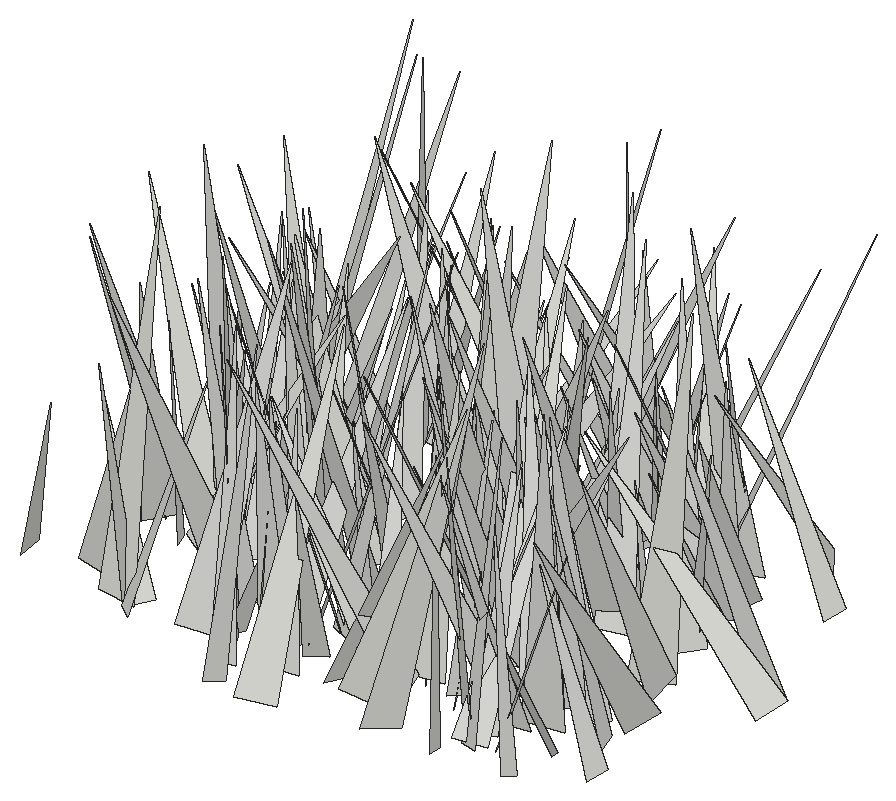
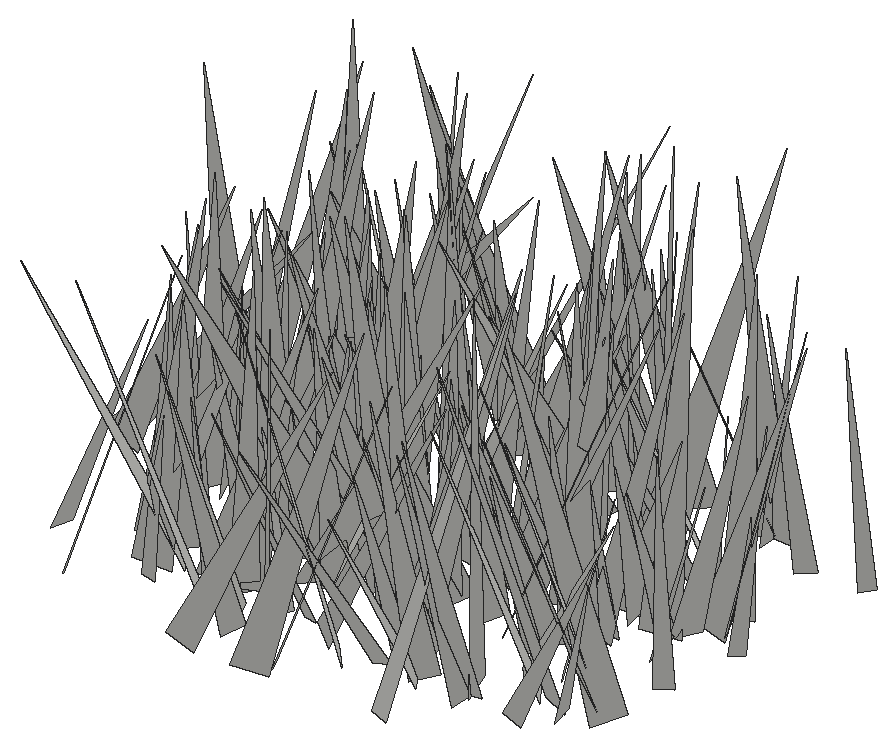
# SketchUp Ruby script. Lengths in inches.
U = 1.inch
M = Sketchup.active_model
def pt(a) = Geom::Point3d.new(a.map { |v| v * U })
def face(e, loops, mat)
  f = e.add_face(loops[0].map { |a| pt(a) })
  loops[1..].each { |l| e.add_face(l.map { |a| pt(a) }).erase! }
  f.material = f.back_material = mat if mat
  f
end
# faces: each face lists its corners as indices into pts; further lists are holes
def faces(e, pts, list, mat = nil) = list.each { |f| face(e, (f[0].is_a?(Array) ? f : [f]).map { |l| l.map { |i| pts[i] } }, mat) }
# xy, xz, yz: faces in a plane at the given z, y or x. An outline is a flat list of corners, or four numbers for a rectangle; further outlines are holes
def ring(l) = l.size == 4 ? [[l[0], l[1]], [l[2], l[1]], [l[2], l[3]], [l[0], l[3]]] : l.each_slice(2).to_a
def flat(e, list, mat, &to3) = list.each { |f| face(e, (f[0].is_a?(Array) ? f : [f]).map { |l| ring(l).map { |u, v| to3.(u, v) } }, mat) }
def xy(e, z, list, mat = nil) = flat(e, list, mat) { |x, y| [x, y, z] }
def xz(e, y, list, mat = nil) = flat(e, list, mat) { |x, z| [x, y, z] }
def yz(e, x, list, mat = nil) = flat(e, list, mat) { |y, z| [x, y, z] }
def lines(e, pts, list) = list.each { |a, b| e.add_line(pt(pts[a]), pt(pts[b])) }
# prism: a flat outline (further loops are holes) pulled along v
def prism(e, loops, v, mat = nil)
  f = face(e, loops, mat); d = Geom::Vector3d.new(v.map { |x| x * U })
  f.pushpull(f.normal.samedirection?(d) ? d.length : -d.length)
end
def box(e, o, s, mat = nil) = prism(e, [[o, [o[0] + s[0], o[1], o[2]], [o[0] + s[0], o[1] + s[1], o[2]], [o[0], o[1] + s[1], o[2]]]], [0, 0, s[2]], mat)
def at(x, y, z, deg = 0) = Geom::Transformation.translation(pt([x, y, z])) * Geom::Transformation.rotation(ORIGIN, Z_AXIS, deg.degrees)
def axes(o, x, y, z) = Geom::Transformation.new([*x, 0, *y, 0, *z, 0, *pt(o).to_a, 1])
def part(name) = M.definitions.add(name)
# library, detail: a bought-in or finely detailed component or shape, given as its bounding box
def library(name, o, s) = part(name).tap { |d| box(d.entities, o, s) }
def detail(e, o, s) = box(e.add_group.entities, o, s)
def put(e, d, t, mat = nil) = e.add_instance(d, t).tap { |i| i.material = mat if mat }
def group(e, t, mat = nil) = e.add_group.tap { |g| g.transformation = t; g.material = mat if mat }.entities
root = M.entities
c1 = part("fur_instance\#9")
p = [[0.8125,0,1.79],[0.67,-0.02,1.48],[0,-0.11,0],[0,0.11,0]]
faces(c1.entities,p,[[0,1,2,3]])
put(root,c1,axes([121.75,413.82,-27.1],[1.49133,-6.04191,1.54576],[-6.23212,-1.50337,0.13646],[-0.23383,1.53405,6.22175]))
put(root,c1,axes([127.07,414.8,-27.1],[-7.35388,-1.92649,0.06127],[-1.88282,7.23164,1.39751],[0.41243,-1.33667,7.47248]))
put(root,c1,axes([123.36,410.6,-27.1],[-3.83392,6.10516,1.11787],[5.9137,3.99214,-1.52073],[1.88436,-0.10697,7.04694]))
put(root,c1,axes([114.97,413.87,-27.1],[-4.71927,-1.33587,1.95814],[-1.09743,5.09822,0.83318],[2.10107,-0.33763,4.83341]))
put(root,c1,axes([122.98,414.57,-27.1],[2.32528,-3.90872,0.2043],[-3.90658,-2.33236,-0.15975],[-0.24182,0.09371,4.54527]))
put(root,c1,axes([130.97,415.68,-27.1],[-7.04471,-1.4589,1.32068],[-0.96261,6.83613,2.41686],[1.71638,-2.15394,6.77607]))
put(root,c1,axes([130.64,411.8125,-27.1],[-5.01766,-1.40088,1.70753],[-1.93126,4.83928,-1.7049],[1.07162,2.16194,4.92267]))
put(root,c1,axes([109.97,414.36,-27.1],[4.41728,-0.60705,0.29796],[-0.51929,-4.30631,-1.07505],[-0.43316,-1.02804,4.32726]))
put(root,c1,axes([121.25,410.86,-27.1],[-5.97598,0.81352,1.54005],[0.17172,5.75229,-2.37225],[1.73323,2.235,5.54496]))
put(root,c1,axes([121.75,414.43,-27.1],[4.45698,-3.93649,1.376],[-3.92382,-4.64074,-0.56675],[-1.41173,0.47074,5.91941]))
put(root,c1,axes([128.1,411.89,-27.1],[7.25129,-2.23194,2.73946],[-2.93898,-7.28136,1.84704],[-1.96177,2.6585,7.35875]))
put(root,c1,axes([121.08,413.58,-27.1],[4.15437,2.45212,1.76514],[2.75663,-4.30471,-0.50784],[-1.23677,-1.35794,4.79727]))
put(root,c1,axes([126.07,413.14,-27.1],[3.27115,-5.93629,2.22387],[-6.24966,-2.60094,2.25],[1.06155,2.98013,6.39355]))
put(root,c1,axes([118,416.32,-27.1],[3.07442,-7.15508,0.96712],[-6.88437,-3.22185,-1.95131],[-2.1762,0.08396,7.5392]))
put(root,c1,axes([122.84,412.96,-27.1],[-0.37436,4.96388,1.61425],[5.21969,0.34743,0.14211],[-0.02763,-1.62026,4.97594]))
put(root,c1,axes([132.09,413.77,-27.1],[4.65437,1.55789,0.49043],[1.62302,-4.57734,-0.86283],[-0.1826,-0.97553,4.83174]))
put(root,c1,axes([136.32,414.03,-27.1],[-4.20728,0.83557,0.99678],[1.00115,4.23485,0.67581],[0.83033,-0.87227,4.23588]))
put(root,c1,axes([130.74,413.6,-27.1],[3.92843,5.06138,3.38638],[5.5366,-4.64662,0.52215],[-2.53598,-2.30413,6.38572]))
put(root,c1,axes([120.65,412.1,-27.1],[0.64289,6.12986,1.03372],[6.0316,-0.86662,1.38779],[-1.50455,-0.85491,6.00521]))
put(root,c1,axes([133.84,412.05,-27.1],[-4.92435,-0.05312,0.24709],[-0.15186,4.47527,-2.06445],[0.20202,2.06935,4.47102]))
put(root,c1,axes([119.71,414.01,-27.1],[4.16125,-1.09144,0.28201],[-1.11074,-4.15389,0.31328],[-0.19241,0.37504,4.29058]))
put(root,c1,axes([112.49,414.71,-27.1],[0.76926,-4.66703,1.07076],[-4.59745,-0.41678,1.48633],[1.33832,1.25083,4.49041]))
put(root,c1,axes([126.06,414.55,-27.1],[-4.18794,0.93567,0.33129],[0.9893,4.05153,1.06324],[0.08071,-1.11073,4.15738]))
put(root,c1,axes([124.67,413.74,-27.1],[6.16079,-1.33707,0.34037],[-1.37023,-6.11166,0.79308],[-0.16154,0.84778,6.25413]))
put(root,c1,axes([132.01,415.01,-27.1],[-1.08629,-5.09453,1.21583],[-5.17343,0.84989,-1.06105],[-0.81738,1.39139,5.09985]))
put(root,c1,axes([115.7,413.76,-27.1],[-3.05082,2.35934,0.28628],[2.37608,3.01778,0.45074],[-0.05159,-0.53147,3.83025]))
put(root,c1,axes([114.69,413.4375,-27.1],[0.76042,7.54721,2.45249],[7.93568,-0.724,-0.23253],[-0.00259,-2.46349,7.58186]))
put(root,c1,axes([135.22,418.04,-27.1],[5.40671,-4.03304,0.21931],[-3.53675,-4.90438,-2.9974],[-1.95061,-2.2864,6.04264]))
put(root,c1,axes([119.75,414.11,-27.1],[4.32475,3.25099,2.86901],[3.37923,-5.06616,0.64681],[-2.71679,-1.12634,5.37159]))
put(root,c1,axes([115.56,412.82,-27.1],[2.99735,3.72962,0.28981],[3.68324,-3.00724,0.60693],[-0.65404,0.15682,4.74613]))
put(root,c1,axes([132.59,415.61,-27.1],[2.16747,-6.96935,1.82134],[-7.20329,-2.08612,0.58967],[0.04123,1.91397,7.27476]))
put(root,c1,axes([131.39,412.8,-27.1],[2.56304,5.03632,1.18387],[4.82189,-2.80423,1.49027],[-1.87495,-0.32715,5.45094]))
put(root,c1,axes([118.48,413.36,-27.1],[-2.56408,6.91655,2.55207],[6.94878,3.17004,-1.60986],[2.46298,-1.74312,7.19872]))
put(root,c1,axes([134.1875,414.28,-27.1],[-5.38862,-5.55187,0.24968],[-4.68183,4.34761,-4.37054],[-2.99434,3.19341,6.38427]))
put(root,c1,axes([118.8125,415.65,-27.1],[-6.63003,0.58928,2.6026],[0.94805,7.03587,0.82207],[2.49439,-1.10786,6.6052]))
put(root,c1,axes([131.35,413.7,-27.1],[-4.05743,3.11883,1.27429],[2.94276,4.25195,-1.03673],[1.64046,0.08657,5.0115]))
put(root,c1,axes([126.52,413.87,-27.1],[-2.91757,4.706,0.99504],[4.75363,2.9987,-0.24403],[0.73452,-0.71423,5.53165]))
put(root,c1,axes([129.02,415.02,-27.1],[3.30079,2.00098,0.99665],[2.11543,-3.37049,-0.23912],[-0.72261,-0.72685,3.85253]))
put(root,c1,axes([122.03,417.01,-27.1],[-4.79453,-5.10071,1.01007],[-5.15614,4.84133,-0.02673],[0.67211,0.75447,7.00029]))
put(root,c1,axes([128.05,417.26,-27.1],[5.66121,2.03663,0.41958],[1.99596,-4.98096,-2.75306],[0.58316,-2.72311,5.34956]))
put(root,c1,axes([135.13,416.07,-27.1],[-4.98874,-1.77944,1.14235],[-1.81158,5.1064,0.04294],[1.09068,0.3424,5.29642]))
put(root,c1,axes([131.25,413.07,-27.1],[-3.49002,4.97532,0.38419],[4.70613,3.43753,-1.76559],[1.65943,0.71499,5.81522]))
put(root,c1,axes([116.8,417.63,-27.1],[-4.19902,-6.23031,2.61813],[-6.01537,4.8505,1.89504],[3.08005,0.97931,7.27031]))
put(root,c1,axes([127.11,415.78,-27.1],[-1.46748,5.77462,2.34569],[6.13429,1.76496,-0.50731],[1.10405,-2.13089,5.93652]))
put(root,c1,axes([126.41,416.12,-27.1],[5.41159,0.09186,1.28906],[0.07062,-5.56242,0.09991],[-1.29039,0.08081,5.41145]))
put(root,c1,axes([132.98,417.5,-27.1],[2.11565,-6.08651,1.80009],[-6.2822,-2.27872,-0.32139],[-0.90548,1.58863,6.43571]))
put(root,c1,axes([116.19,417.57,-27.1],[5.48101,-1.25937,0.85366],[-1.15676,-5.52263,-0.72019],[-0.98826,-0.52035,5.57753]))
put(root,c1,axes([116.03,416.14,-27.1],[3.45283,2.51437,0.03768],[2.48973,-3.40925,-0.65094],[0.3531,-0.54815,4.22141]))
put(root,c1,axes([123.1,416.98,-27.1],[-4.21656,2.08304,0.19454],[2.06998,4.09043,1.06765],[-0.30342,-1.04195,4.58024]))
put(root,c1,axes([128.22,418.82,-27.1],[-3.59271,-3.52154,0.36411],[-3.38524,3.56898,1.11534],[1.03633,-0.55007,4.90559]))
put(root,c1,axes([133.88,417.23,-27.1],[1.42768,-3.34431,1.65268],[-3.54003,-1.77266,-0.52903],[-1.17641,1.27565,3.59761]))
put(root,c1,axes([123.36,418.99,-27.1],[-0.67207,-6.04885,0.74296],[-6.03248,0.76649,0.78356],[0.86591,0.6451,6.03542]))
put(root,c1,axes([129.29,418.52,-27.1],[-0.74587,-6.40704,1.23448],[-6.45249,0.53969,-1.09751],[-0.96927,1.33753,6.35625]))
put(root,c1,axes([112.27,419.03,-27.1],[4.76035,-4.27512,0.72339],[-4.20428,-4.81383,-0.78223],[-1.06017,-0.10597,6.35025]))
put(root,c1,axes([134.24,420.4,-27.1],[6.25747,-1.85529,1.59771],[-1.00282,-5.94215,-2.97253],[-2.23363,-2.52972,5.81052]))
put(root,c1,axes([127.14,415.69,-27.1],[5.31118,5.11176,2.74997],[4.78098,-5.96627,1.85658],[-3.29161,-0.41778,7.13385]))
put(root,c1,axes([129.2,416.97,-27.1],[-7.32876,-0.97242,0.83606],[-1.07916,7.29688,-0.97277],[0.69283,1.07947,7.32872]))
put(root,c1,axes([121.81,419.35,-27.1],[-2.25691,-7.5793,1.44794],[-7.71352,2.17504,-0.63772],[-0.20948,1.56823,7.88243]))
put(root,c1,axes([125.21,418.43,-27.1],[-3.55918,-3.90599,0.48478],[-3.91702,3.45103,-0.95229],[-0.38568,0.99656,5.19785]))
put(root,c1,axes([128.62,415.44,-27.1],[1.86893,4.92203,0.04113],[4.36091,-1.67616,2.42774],[-2.28266,0.8277,4.67176]))
put(root,c1,axes([124.77,419.37,-27.1],[4.05285,-0.43746,0.41546],[-0.3233,-3.95717,-1.01285],[-0.50937,-0.96903,3.94856]))
put(root,c1,axes([122.45,418.25,-27.1],[0.90627,3.33198,1.59944],[3.57947,-1.20149,0.47479],[-0.9207,-1.39138,3.42023]))
put(root,c1,axes([112.03,419.77,-27.1],[-5.14482,-3.13912,1.24988],[-3.04737,5.29445,0.7535],[1.4594,-0.01101,5.97959]))
put(root,c1,axes([113.89,418.13,-27.1],[-3.72029,-1.54775,1.40082],[-1.82397,3.80239,-0.64288],[1.01535,1.15959,3.97778]))
put(root,c1,axes([130.78,417.55,-27.1],[-2.14866,5.91991,1.32548],[6.06222,2.04254,0.70466],[-0.22751,-1.48381,6.25824]))
put(root,c1,axes([122.1875,415.27,-27.1],[6.2923,4.31715,0.79405],[3.75537,-6.01297,2.93303],[-2.27277,2.01685,7.04472]))
put(root,c1,axes([118.12,421.52,-27.1],[-1.88375,-7.99896,1.23534],[-7.80751,2.13018,1.88761],[2.13359,0.73274,7.99805]))
put(root,c1,axes([124.57,419.62,-27.1],[4.01557,-5.25956,2.05629],[-5.53772,-4.16187,0.169],[-1.10676,1.74125,6.61508]))
put(root,c1,axes([122.62,416.42,-27.1],[3.92721,6.27569,0.86047],[6.07775,-4.01843,1.56873],[-1.78486,0.12492,7.23508]))
put(root,c1,axes([125.4375,422.11,-27.1],[4.78768,-6.87101,0.53821],[-6.76798,-4.81092,-1.21319],[-1.30189,-0.25808,8.28619]))
put(root,c1,axes([112.44,420.25,-27.1],[-0.64276,-5.9949,1.38637],[-6.03632,0.34404,-1.31091],[-1.1932,1.48889,5.88502]))
put(root,c1,axes([120.71,416.26,-27.1],[-4.56425,4.1816,0.8559],[3.58274,4.43445,-2.55936],[2.31998,1.37862,5.63629]))
put(root,c1,axes([114.54,418.15,-27.1],[2.28513,5.39499,0.34939],[5.12885,-2.04337,-1.99232],[1.70965,-1.08097,5.50984]))
put(root,c1,axes([110.66,420.98,-27.1],[4.01864,-1.00258,0.99057],[-0.63294,-3.95809,-1.43832],[-1.25928,-1.21004,3.88405]))
put(root,c1,axes([119.65,419.21,-27.1],[-6.31517,-2.67121,2.41272],[-3.08957,6.52254,-0.86542],[1.84694,1.77736,6.80204]))
put(root,c1,axes([127.1,419.68,-27.1],[4.74645,-3.63152,0.20608],[-3.44873,-4.38539,2.15263],[1.15614,1.82746,5.57521]))
put(root,c1,axes([119.5,418.17,-27.1],[-6.71,0.21588,0.88951],[-0.0468,6.49159,-1.92847],[0.91413,1.91692,6.43053]))
put(root,c1,axes([116.85,418.74,-27.1],[-1.85743,4.94831,0.92273],[4.99711,1.93095,-0.29602],[0.60509,-0.75691,5.27714]))
put(root,c1,axes([130.01,423.07,-27.1],[2.00321,-7.73932,0.37509],[-7.71802,-2.02729,-0.61059],[-0.68548,0.20889,7.97102]))
put(root,c1,axes([121.49,420.89,-27.1],[1.52564,-3.34819,0.07276],[-3.07421,-1.36842,1.48995],[1.32851,0.67846,3.36423]))
put(root,c1,axes([127.65,420.69,-27.1],[-2.05605,-4.2865,1.82271],[-4.5186,2.31917,0.35698],[1.13077,1.47345,4.74068]))
put(root,c1,axes([113.77,421.5,-27.1],[1.30407,-7.61557,2.3618],[-7.95747,-1.39423,-0.10194],[-0.50366,2.30972,7.72574]))
put(root,c1,axes([133.57,420.59,-27.1],[-3.8242,6.03816,3.67075],[6.53219,4.61268,-0.78232],[2.69524,-2.61192,7.10435]))
put(root,c1,axes([128.375,420.125,-27.1],[2.97809,2.23148,0.68885],[2.24903,-3.04112,0.12836],[-0.62921,-0.30835,3.71915]))
put(root,c1,axes([128.8,418.32,-27.1],[-3.78371,6.02543,0.57396],[5.96039,3.82698,-0.88298],[1.05307,-0.01122,7.05993]))
put(root,c1,axes([138.27,421.67,-27.1],[-5.02457,3.67244,0.21301],[3.24783,4.25941,3.17608],[-1.72736,-2.67378,5.35216]))
put(root,c1,axes([120.51,421.94,-27.1],[-3.95359,-4.39819,1.62013],[-4.4402,4.19331,0.54823],[1.50116,0.81969,5.8885]))
put(root,c1,axes([133.375,420.91,-27.1],[-3.75742,-0.36081,1.22113],[-0.40687,3.94545,-0.08619],[1.20657,0.20686,3.77372]))
put(root,c1,axes([127.06,423.28,-27.1],[1.34944,-6.66989,1.0863],[-6.57389,-1.5523,-1.36482],[-1.56569,0.76902,6.66676]))
put(root,c1,axes([126.93,420.36,-27.1],[-2.07994,4.49979,1.08625],[4.57933,2.1742,-0.23818],[0.67657,-0.88257,4.95151]))
put(root,c1,axes([127.15,423.63,-27.1],[3.45501,-4.88886,0.26504],[-4.85303,-3.46254,-0.60598],[-0.64754,-0.13474,5.95575]))
put(root,c1,axes([112.99,420.98,-27.1],[-5.78073,2.46703,0.60773],[2.49572,5.79658,0.20851],[0.47643,-0.43109,6.28168]))
put(root,c1,axes([120.31,420.96,-27.1],[-1.88222,6.06948,1.49765],[6.0067,1.32242,2.18977],[-1.73238,-2.00921,5.96542]))
put(root,c1,axes([115.4375,423.01,-27.1],[-1.29627,-6.42722,1.30707],[-6.54569,1.18361,-0.67151],[-0.41416,1.4099,6.52216]))
put(root,c1,axes([114.96,422.69,-27.1],[3.94876,4.2171,2.00571],[4.64379,-3.26946,-2.26834],[0.4919,-2.98768,5.31331]))
put(root,c1,axes([118.19,424.88,-27.1],[-6.16351,-3.9605,0.27898],[-3.73191,5.95492,2.08903],[1.35509,-1.6142,7.02213]))
put(root,c1,axes([126.96,423.53,-27.1],[3.0521,-3.8403,0.46149],[-3.78154,-3.08617,-0.67208],[-0.8129,-0.06212,4.85917]))
put(root,c1,axes([115.87,420.93,-27.1],[-2.49681,4.68547,0.3153],[4.52882,2.308,1.56527],[-1.24213,-1.0033,5.07323]))
put(root,c1,axes([137.68,422.41,-27.1],[-0.80032,5.57612,2.90873],[5.9333,-0.30294,2.21326],[-2.08561,-3.00158,5.18026]))
put(root,c1,axes([117.55,421.87,-27.1],[3.71191,-5.65782,4.04126],[-6.28277,-4.69165,-0.79764],[-2.97818,2.84578,6.7196]))
put(root,c1,axes([128.4,420.99,-27.1],[-3.95695,1.67084,0.9926],[1.45221,4.03835,-1.00857],[1.29152,0.5783,4.17516]))
put(root,c1,axes([119.03,422.3125,-27.1],[-7.40149,0.22253,0.007],[0.22253,7.40149,0.00759],[0.00677,-0.0078,7.40483]))
put(root,c1,axes([115.65,423.8,-27.1],[5.14782,-4.26055,1.16689],[-4.27581,-5.25589,-0.32723],[-1.10966,0.4872,6.67423]))
put(root,c1,axes([126.0625,424.35,-27.1],[7.05622,-1.23215,0.51957],[-1.10047,-6.93599,-1.50315],[-0.75967,-1.39725,7.0035]))
put(root,c1,axes([112.97,422.82,-27.1],[-3.79015,-1.11399,0.60809],[-1.15598,3.82064,-0.20588],[0.52388,0.37109,3.9451]))
put(root,c1,axes([132.7,424.11,-27.1],[-1.98967,-4.65459,1.69235],[-4.24096,2.54317,2.00863],[2.55803,0.59592,4.64644]))
put(root,c1,axes([123.68,423.71,-27.1],[0.0585,-4.06465,0.78718],[-4.11626,0.02739,0.44734],[0.44434,0.78888,4.04038]))
put(root,c1,axes([128.87,424.55,-27.1],[-0.89521,-5.51634,1.09126],[-5.41102,1.14576,1.35291],[1.53027,0.82431,5.42227]))
put(root,c1,axes([113.2,421.76,-27.1],[-3.70619,1.07071,1.22273],[0.63141,3.75399,-1.37341],[1.4976,1.06701,3.605]))
put(root,c1,axes([125.53,424.0625,-27.1],[3.59874,-6.83955,3.08177],[-7.12327,-4.18751,-0.97538],[-2.35281,2.21652,7.66674]))
put(root,c1,axes([123.65,423.3,-27.1],[-2.45983,6.23998,3.07468],[6.83629,2.77173,-0.15592],[1.28687,-2.79677,6.7055]))
put(root,c1,axes([111.18,424.52,-27.1],[0.91273,-4.1627,0.50654],[-4.12867,-0.80133,0.85424],[0.734,0.66898,4.1751]))
put(root,c1,axes([115.26,420.78,-27.1],[-5.60466,1.1961,0.32776],[0.92969,5.05609,-2.5538],[0.82084,2.4404,5.13039]))
put(root,c1,axes([122.8125,423.9,-27.1],[7.01983,-0.71592,2.31882],[-0.6287,-7.39114,-0.37866],[-2.34397,-0.1616,7.04608]))
put(root,c1,axes([133.1,426.07,-27.1],[2.61621,-5.42084,0.25429],[-5.22177,-2.59146,-1.52055],[-1.47757,-0.43991,5.82391]))
put(root,c1,axes([134.76,424.09,-27.1],[-1.27388,-3.61865,0.59779],[-3.46584,0.98064,-1.44951],[-1.19998,1.0092,3.55195]))
put(root,c1,axes([122.98,421.62,-27.1],[-0.78819,5.89997,0.04998],[5.7265,0.75282,1.4401],[-1.42105,-0.23877,5.77555]))
put(root,c1,axes([116.57,423.01,-27.1],[-1.7521,4.37342,1.24469],[4.49457,1.86786,-0.23622],[0.6891,-1.06311,4.7054]))
put(root,c1,axes([133.18,423.125,-27.1],[-6.12251,3.37612,2.03098],[3.42132,6.417,-0.35327],[1.95387,-0.65732,6.98272]))
put(root,c1,axes([121.59,424.05,-27.1],[-0.9402,5.50023,2.63792],[6.09336,0.97222,0.14463],[0.28664,-2.62629,5.57814]))
put(root,c1,axes([120.91,423.99,-27.1],[4.20762,-3.32651,0.12048],[-3.15177,-3.91891,1.86887],[1.07075,1.53645,5.02763]))
put(root,c1,axes([127.08,421.95,-27.1],[2.4518,5.85296,0.01413],[5.81055,-2.43218,-0.76857],[0.70347,-0.30989,6.29903]))
put(root,c1,axes([129.95,424.76,-27.1],[-0.88602,-4.48963,1.06047],[-4.46813,0.56653,-1.33464],[-1.14769,1.26043,4.37728]))
put(root,c1,axes([116.01,423.2,-27.1],[4.17653,-0.25853,0.87813],[-0.4857,-4.1025,1.10224],[-0.77592,1.17643,4.03674]))
put(root,c1,axes([132.71,422.75,-27.1],[-5.22043,-0.84385,1.05571],[-1.17009,4.93002,-1.84535],[0.67639,2.01552,4.95577]))
put(root,c1,axes([130.25,422.59,-27.1],[-1.2461,7.24945,1.28302],[7.36015,1.19663,0.38699],[-0.1701,-1.32928,7.34558]))
put(root,c1,axes([126.83,423.125,-27.1],[-3.66348,3.88372,0.60062],[3.90017,3.69385,-0.09601],[0.48235,-0.37054,5.33808]))
put(root,c1,axes([130.51,424.58,-27.1],[4.15283,1.56186,1.94961],[1.7605,-4.5132,-0.13443],[-1.7723,-0.82343,4.43479]))
put(root,c1,axes([132.78,427.03,-27.1],[4.609,-3.3139,0.05026],[-3.15306,-4.41083,-1.68231],[-1.0211,-1.33793,5.42168]))
put(root,c1,axes([131.3,423.52,-27.1],[-1.57636,3.66287,0.67143],[3.67727,1.64614,-0.34684],[0.58749,-0.47537,3.97256]))
put(root,c1,axes([123.48,424.95,-27.1],[4.4628,-4.8312,0.78242],[-4.8199,-4.15484,1.83716],[0.84924,1.80724,6.31521]))
put(root,c1,axes([124.81,424.97,-27.1],[3.82808,-2.96393,0.87418],[-3.08142,-3.76593,0.72521],[-0.23226,1.11183,4.78677]))
put(root,c1,axes([127.22,425.08,-27.1],[3.70956,-2.15387,1.10856],[-2.28011,-3.78925,0.26761],[-0.81802,0.79458,4.28116]))
put(root,c1,axes([121.86,424.77,-27.1],[-3.05036,2.77962,1.08054],[2.93347,3.07501,0.37088],[0.53722,-1.00823,4.11016]))
put(root,c1,axes([131.99,427.41,-27.1],[-3.10911,-5.59083,0.18925],[-5.58666,3.11434,0.22319],[0.28707,0.05678,6.39328]))
put(root,c1,axes([125.95,426.3,-27.1],[-7.5943,2.08618,0.38061],[2.11361,7.33132,1.9887],[-0.17228,-2.01745,7.62041]))
put(root,c1,axes([114.55,426.1,-27.1],[-3.02688,-2.08558,0.64094],[-2.07151,3.09116,0.27563],[0.68504,0.13224,3.66547]))
put(root,c1,axes([111.27,427.59,-27.1],[2.01455,-7.63294,0.11302],[-6.59973,-1.68273,3.99311],[3.83642,1.11337,6.80994]))
put(root,c1,axes([120.86,426.69,-27.1],[-6.83352,3.26319,2.339],[3.80782,6.73136,1.73366],[1.27275,-2.61852,7.37155]))
put(root,c1,axes([128.625,424.63,-27.1],[-5.59489,5.13542,2.2708],[5.22691,5.9344,-0.54239],[2.05147,-1.11455,7.57503]))
put(root,c1,axes([116.65,424.29,-27.1],[5.33264,0.16428,1.51785],[-0.27785,-5.31816,1.55174],[-1.50122,1.56784,5.10452]))
put(root,c1,axes([119.16,424.37,-27.1],[-5.25856,3.05312,1.43062],[2.8843,5.44607,-1.02073],[1.74617,0.1987,5.99435]))
put(root,c1,axes([124.99,426.01,-27.1],[3.66382,-3.28739,1.57998],[-3.52995,-3.75957,0.36325],[-0.918,1.33625,4.90903]))
put(root,c1,axes([127.2,428.11,-27.1],[4.74802,-2.11154,0.82126],[-1.70244,-4.58339,-1.94189],[-1.49491,-1.48682,4.81989]))
put(root,c1,axes([122.82,424.59,-27.1],[1.506,6.6666,0.93752],[6.04421,-0.91584,-3.19677],[2.9648,-1.51928,6.04088]))
put(root,c1,axes([125.47,425.74,-27.1],[-5.46904,-3.01802,0.13387],[-2.92547,5.22183,-1.79189],[-0.75368,1.63119,5.98398]))
put(root,c1,axes([121.11,426.52,-27.1],[0.6303,-6.24139,2.24897],[-6.57772,-0.29373,1.02832],[0.86396,2.31708,6.18828]))
put(root,c1,axes([122.41,425.58,-27.1],[-3.47776,6.78239,3.15196],[7.08859,4.09761,-0.99596],[2.38486,-2.28893,7.55669]))
put(root,c1,axes([128.91,428.3,-27.1],[3.32641,-4.64571,1.36805],[-4.19977,-3.59363,-1.99171],[-2.41165,-0.14974,5.35544]))
put(root,c1,axes([116.39,425.45,-27.1],[-0.0874,4.08723,0.80677],[4.1529,0.14964,-0.30818],[0.33125,-0.79758,4.07653]))
put(root,c1,axes([115.68,426.92,-27.1],[-2.7303,-2.91554,0.15676],[-2.8364,2.59761,-1.08937],[-0.69267,0.85529,3.84294]))
put(root,c1,axes([131.625,427.54,-27.1],[0.51611,-4.80053,1.29544],[-4.96034,-0.40702,0.46794],[0.34389,1.33374,4.80546]))
put(root,c1,axes([123.13,424.66,-27.1],[-3.56356,5.20391,0.71647],[5.00613,3.62664,-1.4419],[1.59144,0.24443,6.14008]))
put(root,c1,axes([125.91,424.35,-27.1],[7.47799,-1.52657,1.95795],[-2.25093,-6.79047,3.30259],[-1.04752,3.69369,6.88067]))
put(root,c1,axes([125.23,428.54,-27.1],[4.19489,0.81761,0.41517],[0.91291,-3.90671,-1.53042],[-0.08632,-1.58339,3.99042]))
put(root,c1,axes([133.32,431.36,-27.1],[-4.76497,-3.93422,0.44703],[-3.2824,4.31602,2.99679],[2.21445,-2.06803,5.40391]))
put(root,c1,axes([127.37,428.4375,-27.1],[5.69628,-2.00129,2.37758],[-1.98509,-6.1627,-0.4314],[-2.39112,0.34864,6.02217]))
put(root,c1,axes([131.26,428.88,-27.1],[0.92373,-7.0899,2.33425],[-7.39568,-1.18748,-0.68009],[-1.00963,2.21177,7.11741]))
put(root,c1,axes([130.72,429.74,-27.1],[-2.364,-4.99525,1.36106],[-4.8414,2.66304,1.36474],[1.83462,0.59091,5.35523]))
put(root,c1,axes([135.64,428.56,-27.1],[-5.10669,0.68056,0.36828],[0.71376,5.09217,0.48729],[0.29888,-0.53268,5.12875]))
put(root,c1,axes([119.1875,427.65,-27.1],[4.30125,1.72732,0.68489],[1.69718,-4.35514,0.32517],[-0.75649,0.05042,4.6237]))
put(root,c1,axes([130.95,427.08,-27.1],[-4.49131,4.50007,0.95246],[4.50728,4.57122,-0.34355],[0.91773,-0.42777,6.34858]))
put(root,c1,axes([113.27,425.9,-27.1],[5.00071,5.94343,0.88428],[5.7504,-5.06729,1.53914],[-1.74336,0.3341,7.61331]))
put(root,c1,axes([123.21,429.07,-27.1],[-3.40667,-4.88664,0.79026],[-4.79108,3.01371,-2.01797],[-1.2447,1.77411,5.60468]))
put(root,c1,axes([116.49,428.66,-27.1],[7.01213,2.59998,3.36264],[2.81322,-7.70163,0.08845],[-3.18638,-1.07803,7.47811]))
put(root,c1,axes([117.9,432.51,-27.1],[-4.53794,-6.8341,0.16977],[-6.57814,4.42074,2.12406],[1.86058,-1.03861,7.92377]))
put(root,c1,axes([129.11,428.3,-27.1],[-3.597,-0.64897,1.74683],[-0.97146,3.89365,-0.55385],[1.59023,0.91068,3.61287]))
put(root,c1,axes([118.375,429.26,-27.1],[4.08731,-3.32744,0.79787],[-3.41978,-4.01464,0.77613],[-0.11643,1.10699,5.21302]))
put(root,c1,axes([114.38,427.6,-27.1],[4.71146,3.59222,0.48874],[3.58656,-4.73541,0.23065],[-0.52868,-0.11206,5.92019]))
put(root,c1,axes([119.79,428.67,-27.1],[-0.91828,3.53646,1.4047],[3.57282,1.29857,-0.93362],[1.30946,-1.06309,3.53244]))
put(root,c1,axes([112.8,428.35,-27.1],[-3.94683,-0.00707,0.27926],[-0.08275,3.80753,-1.07302],[0.26682,1.07619,3.79817]))
put(root,c1,axes([124.25,428.5,-27.1],[2.1149,3.97719,0.39309],[3.90996,-1.96694,-1.13523],[0.82754,-0.87089,4.35914]))
put(root,c1,axes([114.02,429.72,-27.1],[-0.24742,-3.68689,1.2628],[-3.55064,-0.30834,-1.59591],[-1.60648,1.24932,3.33279]))
put(root,c1,axes([113.45,427.92,-27.1],[3.5873,6.66463,1.07182],[6.75002,-3.55215,-0.50434],[-0.05834,-1.18311,7.55193]))
put(root,c1,axes([123.16,431.97,-27.1],[-4.86193,-2.9811,0.43497],[-2.74592,4.72474,1.68858],[1.2394,-1.22654,5.44739]))
put(root,c1,axes([126.58,429.48,-27.1],[4.75078,2.28793,0.55209],[2.32197,-4.75936,-0.25743],[-0.38451,-0.47246,5.26671]))
put(root,c1,axes([116.26,429.79,-27.1],[4.91416,0.05831,0.74386],[0.02898,-4.96646,0.19783],[-0.74558,0.19125,4.91052]))
put(root,c1,axes([123.64,432.78,-27.1],[3.27903,-5.74844,0.73311],[-5.41958,-3.34021,-1.9507],[-2.05188,-0.36394,6.32387]))
put(root,c1,axes([130.66,427.6875,-27.1],[5.97415,4.42308,0.10738],[4.35531,-5.91092,1.16532],[-0.77872,0.87356,7.3414]))
put(root,c1,axes([112.5625,426.98,-27.1],[3.79972,6.90357,0.39781],[6.61789,-3.76205,2.07507],[-2.00527,0.66563,7.60206]))
put(root,c1,axes([126.88,432.72,-27.1],[0.00181,-5.98408,0.19016],[-5.68264,-0.06159,-1.88392],[-1.88493,0.17992,5.67979]))
put(root,c1,axes([116.4,429.27,-27.1],[-0.03084,5.75903,1.17934],[5.85206,0.14189,-0.53988],[0.55736,-1.17118,5.73375]))
put(root,c1,axes([127.26,430.53,-27.1],[5.75926,3.61485,0.22209],[3.58079,-5.62103,-1.36658],[0.54262,-1.27375,6.66098]))
put(root,c1,axes([125.03,430.0625,-27.1],[-5.7993,-3.05465,2.69516],[-3.68736,5.92923,-1.21419],[1.7315,2.39584,6.44116]))
put(root,c1,axes([120.21,429.4,-27.1],[1.05381,5.0713,0.10966],[4.76326,-0.95083,-1.80217],[1.74396,-0.4674,4.856]))
put(root,c1,axes([118.52,429.54,-27.1],[3.43862,2.40363,0.16823],[2.31203,-3.37399,0.94893],[-0.67841,0.6845,4.08669]))
put(root,c1,axes([121.77,429.89,-27.1],[5.53821,4.98185,1.27941],[5.04776,-5.62536,0.05401],[-0.98782,-0.81487,7.449]))
put(root,c1,axes([125.91,430.85,-27.1],[4.66394,-1.20705,1.00362],[-1.36601,-4.67089,0.73033],[-0.77347,0.97077,4.76192]))
